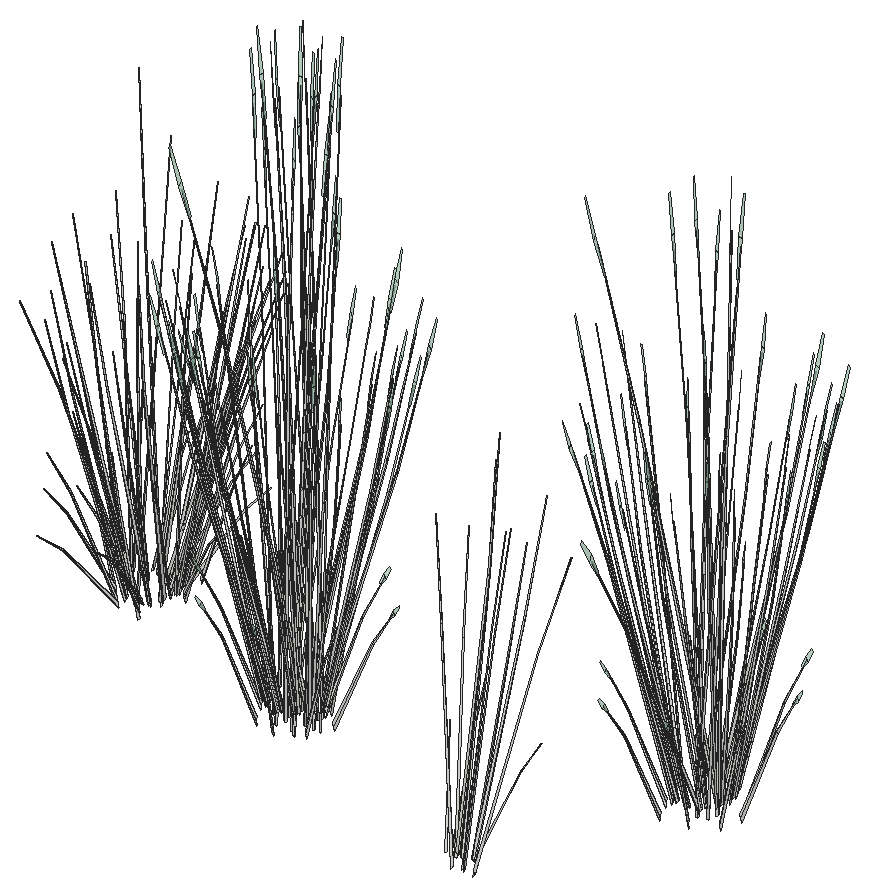
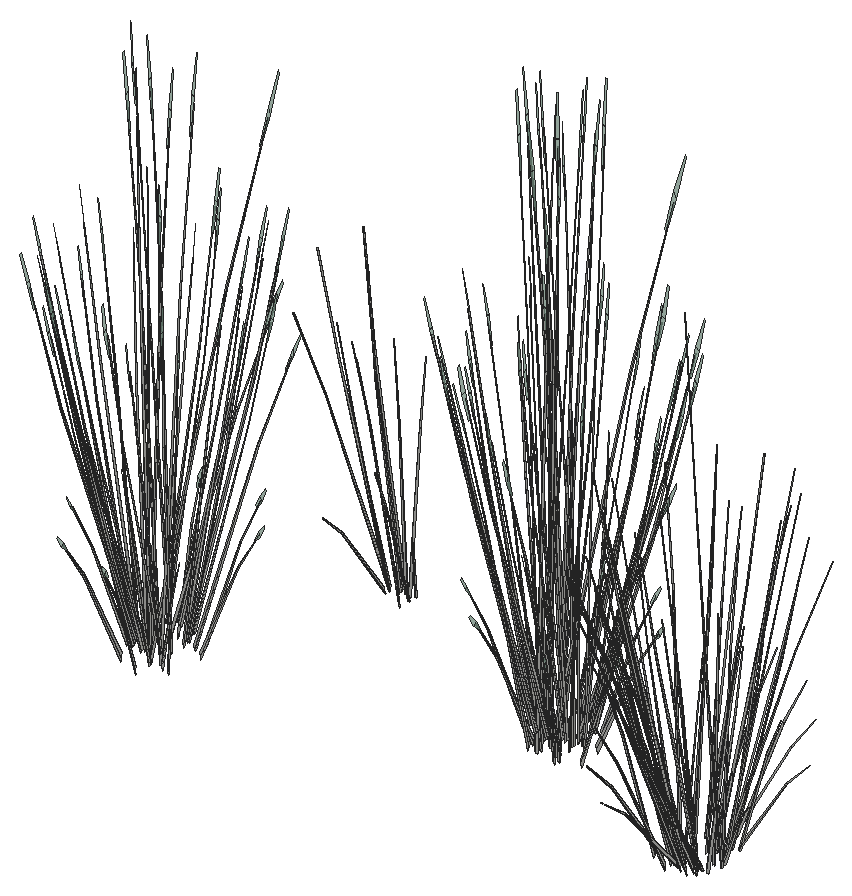
# SketchUp Ruby script. Lengths in inches.
U = 1.inch
M = Sketchup.active_model
def pt(a) = Geom::Point3d.new(a.map { |v| v * U })
def face(e, loops, mat)
  f = e.add_face(loops[0].map { |a| pt(a) })
  loops[1..].each { |l| e.add_face(l.map { |a| pt(a) }).erase! }
  f.material = f.back_material = mat if mat
  f
end
# faces: each face lists its corners as indices into pts; further lists are holes
def faces(e, pts, list, mat = nil) = list.each { |f| face(e, (f[0].is_a?(Array) ? f : [f]).map { |l| l.map { |i| pts[i] } }, mat) }
# xy, xz, yz: faces in a plane at the given z, y or x. An outline is a flat list of corners, or four numbers for a rectangle; further outlines are holes
def ring(l) = l.size == 4 ? [[l[0], l[1]], [l[2], l[1]], [l[2], l[3]], [l[0], l[3]]] : l.each_slice(2).to_a
def flat(e, list, mat, &to3) = list.each { |f| face(e, (f[0].is_a?(Array) ? f : [f]).map { |l| ring(l).map { |u, v| to3.(u, v) } }, mat) }
def xy(e, z, list, mat = nil) = flat(e, list, mat) { |x, y| [x, y, z] }
def xz(e, y, list, mat = nil) = flat(e, list, mat) { |x, z| [x, y, z] }
def yz(e, x, list, mat = nil) = flat(e, list, mat) { |y, z| [x, y, z] }
def lines(e, pts, list) = list.each { |a, b| e.add_line(pt(pts[a]), pt(pts[b])) }
# prism: a flat outline (further loops are holes) pulled along v
def prism(e, loops, v, mat = nil)
  f = face(e, loops, mat); d = Geom::Vector3d.new(v.map { |x| x * U })
  f.pushpull(f.normal.samedirection?(d) ? d.length : -d.length)
end
def box(e, o, s, mat = nil) = prism(e, [[o, [o[0] + s[0], o[1], o[2]], [o[0] + s[0], o[1] + s[1], o[2]], [o[0], o[1] + s[1], o[2]]]], [0, 0, s[2]], mat)
def at(x, y, z, deg = 0) = Geom::Transformation.translation(pt([x, y, z])) * Geom::Transformation.rotation(ORIGIN, Z_AXIS, deg.degrees)
def axes(o, x, y, z) = Geom::Transformation.new([*x, 0, *y, 0, *z, 0, *pt(o).to_a, 1])
def part(name) = M.definitions.add(name)
# library, detail: a bought-in or finely detailed component or shape, given as its bounding box
def library(name, o, s) = part(name).tap { |d| box(d.entities, o, s) }
def detail(e, o, s) = box(e.add_group.entities, o, s)
def put(e, d, t, mat = nil) = e.add_instance(d, t).tap { |i| i.material = mat if mat }
def group(e, t, mat = nil) = e.add_group.tap { |g| g.transformation = t; g.material = mat if mat }.entities
root = M.entities
M.materials.add("LightPink_Translucent").color = [175, 214, 192]
M.materials["LightPink_Translucent"].alpha = 0.75
c1 = part("blade")
p = [[2.15,0.21,22],[0,0.17,0],[0.09,0.45,0],[2.18,0.31,22],[2.29,0.31,22],[0.38,0.45,0],
  [2.48,0.24,33],[2.49,0.24,33],[2.48,0.22,33]]
faces(c1.entities,p,[[0,1,2,3],[4,5,2,3],[6,3,4,7],[8,0,3,6]])
c2 = part("blade with seeds\#1")
put(c2.entities,c1,at(0,0,0))
c3 = part("seeds")
p = [[0.3,-0.1,1.38],[-0.01,-0.03,1.59],[-0.01,-0.03,0.03],[0.14,-0.07,-0.07],[0.29,-0.03,3],[0.15,0.01,3.11]]
faces(c3.entities,p,[[0,1,2,3],[1,0,4,5]],"LightPink_Translucent")
c4 = part("blade with seeds")
put(c4.entities,c1,at(0,0,0))
put(c4.entities,c3,axes([2.4,0.25,30.99],[1.5799,-0.05474,1.17369],[-0.12525,1.92788,0.29478],[-0.07173,-0.02425,1.56792]))
put(root,c2,axes([484.5,550.33,139.9],[0.09256,-0.13097,1.40588],[0.38832,0.27104,0.11368],[-0.17518,0.16893,0.601]))
put(root,c2,axes([484.61,551.07,140.43],[-0.33637,0.20062,-0.29052],[-0.31842,-0.22908,0.37506],[-0.04845,0.11639,0.71765]))
put(root,c2,axes([483.45,551.01,140.59],[-0.01236,0.0754,1.43516],[0.35069,0.26232,-0.22697],[-0.09181,0.12405,0.1151]))
put(root,c2,axes([484.57,550.84,141.15],[0.54637,0.01888,-0.11073],[-0.01493,0.35746,-0.6146],[-0.03795,0.13767,0.93387]))
put(root,c2,axes([485.58,551.24,140.85],[0.48648,-0.17741,-0.09976],[0.23906,0.31487,-0.55369],[0.06419,0.13269,0.84132]))
put(root,c2,axes([484.94,550.98,140.82],[0.35588,0.25603,-0.4653],[-0.37594,0.22422,-0.36041],[-0.05415,0.13008,0.89031]))
put(root,c2,axes([486.28,550.55,139.9],[-0.11364,-0.12234,1.40588],[0.52511,-0.103,0.11368],[0.11868,0.19206,0.601]))
put(root,c2,axes([485.78,551.43,140.43],[-0.14987,0.29303,-0.29052],[-0.43725,-0.08547,0.37506],[0.04009,0.11798,0.71765]))
put(root,c2,axes([485.35,550.61,139.9],[-0.01217,-0.14625,1.40588],[0.52737,0.09702,0.11368],[-0.03262,0.20842,0.601]))
put(root,c2,axes([483.41,551.79,140.58],[0.0564,-0.02301,1.45516],[0.46615,0.15302,-0.1375],[-0.01095,0.12741,0.25751]))
put(root,c2,axes([485.47,551.95,140.59],[0.06302,0.06136,1.43516],[0.50855,0.02411,-0.22697],[0.05114,0.13532,0.1151]))
put(root,c2,axes([484.65,551.36,139.48],[0.01092,-0.19671,1.26617],[0.49126,0.1039,0.17497],[-0.04257,0.20964,0.59789]))
put(root,c4,axes([463.59,558.34,141.8],[-0.22811,-0.3621,-0.64651],[0.46957,-0.2018,0.07802],[-0.05334,-0.17496,0.91455]))
put(root,c4,axes([464.54,558.7,141.8],[0.01244,-0.41193,-0.64651],[0.52368,0.02767,0.07802],[0.05527,-0.17451,0.91455]))
put(root,c4,axes([463.63,558.04,141.38],[0.14409,-0.34247,-0.32227],[0.42037,0.09989,0.41605],[-0.03855,-0.13788,0.79608]))
put(root,c4,axes([463.42,558.27,141.52],[-0.46982,-0.11164,-0.465],[0.16104,-0.38276,-0.36018],[-0.04308,-0.1541,0.88973]))
put(root,c4,axes([463.71,557.3125,139.78],[0.06131,0.25968,1.04523],[-0.34012,-0.14383,0.76796],[0.0366,-0.13297,0.23022]))
put(root,c4,axes([464.43,558.56,141.52],[-0.34214,-0.29922,-0.465],[0.36143,-0.26205,-0.36018],[0.05206,-0.15203,0.88973]))
put(root,c4,axes([464.76,558.45,141.38],[0.32338,-0.23447,-0.32227],[0.30612,0.26773,0.41605],[0.04658,-0.13603,0.79608]))
put(root,c4,axes([461.96,557.625,139.78],[0.24931,0.155,1.04523],[-0.36309,0.09317,0.76796],[-0.07769,-0.11912,0.23022]))
put(root,c4,axes([462.5625,558.45,141.8],[-0.40754,-0.21525,-0.64651],[0.28963,-0.37719,0.07802],[-0.14765,-0.12852,0.91455]))
put(root,c4,axes([462.42,558.16,141.38],[-0.07382,-0.3587,-0.32227],[0.42197,-0.09472,0.41605],[-0.11334,-0.10279,0.79608]))
put(root,c4,axes([462.37,558.46,141.52],[-0.47162,0.10586,-0.465],[-0.0825,-0.4009,-0.36018],[-0.12667,-0.11489,0.88973]))
put(root,c4,axes([465.16,559.41,141.8],[0.24965,-0.35138,-0.64651],[0.43748,0.24972,0.07802],[0.14906,-0.12731,0.91455]))
put(root,c4,axes([465.14,559.25,141.52],[-0.12278,-0.40663,-0.465],[0.46497,-0.07113,-0.36018],[0.13325,-0.10922,0.88973]))
put(root,c4,axes([463.54,560.88,140.29],[0.41302,0.17958,1.37647],[-0.40462,0.38687,0.54432],[-0.18124,-0.22929,1.15394]))
put(root,c4,axes([465.71,558.44,139.78],[-0.15919,0.2267,1.04523],[-0.13683,-0.30457,0.76796],[0.13148,-0.07632,0.23022]))
put(root,c4,axes([465.49,559.29,141.38],[0.41603,-0.06364,-0.32227],[0.10985,0.36383,0.41605],[0.11922,-0.09772,0.79608]))
put(root,c4,axes([461.44,558.79,141.38],[-0.27194,-0.27882,-0.32227],[0.31051,-0.26394,0.41605],[-0.15777,-0.04016,0.79608]))
put(root,c4,axes([461.73,558.98,141.8],[-0.47777,-0.01072,-0.64651],[0.03209,-0.45152,0.07802],[-0.2024,-0.04765,0.91455]))
put(root,c4,axes([461.57,559.07,141.52],[-0.34704,0.29499,-0.465],[-0.30393,-0.31162,-0.36018],[-0.17633,-0.04488,0.88973]))
put(root,c4,axes([460.79,559.46,139.78],[0.30513,-0.03187,1.04523],[-0.19355,0.28077,0.76796],[-0.15079,-0.04212,0.23022]))
put(root,c4,axes([462.95,559.72,139.74],[-0.519,0.02749,0.40713],[-0.04694,-0.45634,-0.19594],[0.09291,-0.04625,1.30716]))
put(root,c4,axes([461.61,560.05,139.52],[0,0.44533,0.45182],[-0.53472,0,0],[0,-0.10143,1.43328]))
put(root,c4,axes([465.36,560.15,141.52],[0.12948,-0.40508,-0.465],[0.44393,0.13885,-0.36018],[0.17873,-0.03714,0.88973]))
put(root,c4,axes([462.82,560.28,139.74],[-0.23189,0.40128,0.40713],[-0.48183,-0.19312,-0.19594],[0,-0.0925,1.30716]))
put(root,c4,axes([464.4,558.74,139.52],[-0.44731,-0.22267,0.45182],[0.26736,-0.39927,0],[0.10188,0.05071,1.43328]))
put(root,c4,axes([465.28,560.3,141.8],[0.41997,-0.19668,-0.64651],[0.23405,0.40486,0.07802],[0.20292,-0.04599,0.91455]))
put(root,c4,axes([462.7,558.9375,139.52],[-0.13807,0.44258,0.16054],[-0.50524,-0.12525,0.31929],[0.08728,-0.00216,1.4597]))
put(root,c4,axes([463.57,559.53,139.74],[-0.28711,-0.37379,0.40713],[0.43489,-0.26322,-0.19594],[0.09291,0.04625,1.30716]))
put(root,c4,axes([462.66,561.22,139.52],[0.51358,-0.1182,0.16054],[0.12682,0.43988,0.31929],[-0.0458,-0.06409,1.4597]))
put(root,c4,axes([465.63,560.34,141.38],[0.3972,0.12423,-0.32227],[-0.11585,0.36244,0.41605],[0.15992,-0.03323,0.79608]))
put(root,c4,axes([460.96,559.76,141.38],[-0.3972,-0.12423,-0.32227],[0.11585,-0.36244,0.41605],[-0.15992,0.03323,0.79608]))
put(root,c4,axes([464.23,558.96,139.52],[-0.51358,0.1182,0.16054],[-0.12682,-0.43988,0.31929],[0.0458,0.06409,1.4597]))
put(root,c2,axes([445.41,563.42,140.68],[-0.05804,-0.06898,1.43516],[-0.35603,0.0883,-0.22697],[-0.0675,-0.17309,0.1151]))
put(root,c4,axes([464.18,561.24,139.52],[0.13807,-0.44258,0.16054],[0.50524,0.12525,0.31929],[-0.08728,0.00216,1.4597]))
put(root,c4,axes([462.17,559.7,140.31],[0.13585,-0.06442,1.61128],[0.04685,0.4498,0.1261],[-0.29426,0.05969,0.57588]))
put(root,c4,axes([464.97,560.11,139.52],[-0.37551,-0.32439,0.16054],[0.37842,-0.31463,0.31929],[-0.04147,0.06625,1.4597]))
put(root,c4,axes([466.47,560.41,139.78],[-0.2953,0.07352,1.04523],[0.139,-0.30384,0.76796],[0.15666,0.02079,0.23022]))
put(root,c2,axes([446.97,563.78,140.68],[-0.03336,0.04495,1.45516],[-0.35758,-0.09833,-0.1375],[-0.02285,-0.17707,0.25751]))
put(root,c4,axes([462.49,561.44,139.52],[0.44731,0.22267,0.45182],[-0.26736,0.39927,0],[-0.10188,-0.05071,1.43328]))
put(root,c2,axes([445.43,565.64,139.99],[0.00863,0.2062,1.40588],[-0.37404,-0.13679,0.11368],[0.02314,-0.29386,0.601]))
put(root,c4,axes([464.07,559.9,139.74],[0.23189,-0.40128,0.40713],[0.48183,0.19312,-0.19594],[0,0.0925,1.30716]))
put(root,c4,axes([461.24,559.94,141.52],[-0.12948,0.40508,-0.465],[-0.44393,-0.13885,-0.36018],[-0.17873,0.03714,0.88973]))
put(root,c4,axes([493.37,566.32,140.21],[0.06442,0.13585,1.61128],[-0.4498,0.04685,0.1261],[-0.05969,-0.29426,0.57588]))
put(root,c2,axes([445.81,564.52,140.53],[0.1063,-0.41315,-0.29052],[0.31012,0.1205,0.37506],[-0.02844,-0.16634,0.71765]))
put(root,c4,axes([465.28,560.125,139.52],[0,-0.44533,0.45182],[0.53472,0,0],[0,0.10143,1.43328]))
put(root,c4,axes([463.94,560.46,139.74],[0.519,-0.02749,0.40713],[0.04694,0.45634,-0.19594],[-0.09291,0.04625,1.30716]))
put(root,c4,axes([494.09,565.875,141.7],[0.01072,-0.47777,-0.64651],[0.45152,0.03209,0.07802],[0.04765,-0.2024,0.91455]))
put(root,c2,axes([446.43,564.9,140.68],[-0.00644,-0.10664,1.43516],[-0.29603,-0.29251,-0.22697],[0.03908,-0.18969,0.1151]))
put(root,c4,axes([493.3125,565.11,141.29],[0.12423,-0.3972,-0.32227],[0.36244,0.11585,0.41605],[-0.03323,-0.15992,0.79608]))
put(root,c4,axes([493.125,565.38,141.43],[-0.40508,-0.12948,-0.465],[0.13885,-0.44393,-0.36018],[-0.03714,-0.17873,0.88973]))
put(root,c2,axes([445.95,564.78,140.94],[-0.34504,0.25013,-0.09976],[-0.16956,-0.44394,-0.55369],[-0.04552,-0.18708,0.84132]))
put(root,c2,axes([446.66,565.34,140.94],[-0.38751,-0.02662,-0.09976],[0.01059,-0.50399,-0.55369],[0.02692,-0.19411,0.84132]))
put(root,c4,axes([494,565.71,141.43],[-0.29499,-0.34704,-0.465],[0.31162,-0.30393,-0.36018],[0.04488,-0.17633,0.88973]))
put(root,c2,axes([445.04,563.67,140.68],[-0.00289,0.06493,1.45516],[-0.31009,0.26964,-0.1375],[-0.10196,-0.10828,0.25751]))
put(root,c2,axes([444.92,564.67,140.53],[-0.05446,-0.43273,-0.29052],[0.31131,-0.11427,0.37506],[-0.08362,-0.12401,0.71765]))
put(root,c2,axes([446.64,565.02,140.53],[0.23857,-0.28286,-0.29052],[0.22584,0.32298,0.37506],[0.03436,-0.1641,0.71765]))
put(root,c4,axes([464.86,561.12,141.8],[0.47777,0.01072,-0.64651],[-0.03209,0.45152,0.07802],[0.2024,0.04765,0.91455]))
put(root,c4,axes([464.33,561.48,139.52],[0.44731,-0.22267,0.45182],[0.26736,0.39927,0],[-0.10188,0.05071,1.43328]))
put(root,c4,axes([491.39,564.5,139.6875],[0.20183,0.19918,1.04523],[-0.31952,0.0786,0.76796],[-0.05721,-0.14394,0.23022]))
put(root,c2,axes([446.03,566.03,139.99],[-0.06565,0.18466,1.40588],[-0.27542,-0.38215,0.11368],[0.12424,-0.23818,0.601]))
put(root,c4,axes([494.28,565.59,141.29],[0.27882,-0.27194,-0.32227],[0.26394,0.31051,0.41605],[0.04016,-0.15777,0.79608]))
put(root,c4,axes([492.27,565.25,141.29],[-0.06364,-0.41603,-0.32227],[0.36383,-0.10985,0.41605],[-0.09772,-0.11922,0.79608]))
put(root,c4,axes([460.36,561.68,139.78],[0.19918,-0.20183,1.04523],[0.0786,0.31952,0.76796],[-0.14394,0.05721,0.23022]))
put(root,c4,axes([465.15,561.3,141.38],[0.27194,0.27882,-0.32227],[-0.31051,0.26394,0.41605],[0.15777,0.04016,0.79608]))
put(root,c4,axes([461.11,560.8,141.38],[-0.41603,0.06364,-0.32227],[-0.10985,-0.36383,0.41605],[-0.11922,0.09772,0.79608]))
put(root,c4,axes([493.61,564.93,139.6875],[0.03187,0.30513,1.04523],[-0.28077,-0.19355,0.76796],[0.04212,-0.15079,0.23022]))
put(root,c2,axes([446.67,564.17,140.04],[-0.32031,0.09515,-0.02864],[-0.07364,-0.44972,-0.12987],[0.02031,-0.09391,0.42837]))
put(root,c2,axes([445.13,564.8,140.94],[-0.21011,0.45986,-0.09976],[-0.30427,-0.26493,-0.55369],[-0.10577,-0.12992,0.84132]))
put(root,c4,axes([464.83,561.46,139.78],[-0.2691,-0.12805,1.04523],[0.34747,-0.13011,0.76796],[0.09372,0.11021,0.23022]))
put(root,c4,axes([492.22,565.59,141.43],[-0.40663,0.12278,-0.465],[-0.07113,-0.46497,-0.36018],[-0.10922,-0.13325,0.88973]))
put(root,c2,axes([447.09,566.33,140.94],[-0.32616,-0.29624,-0.09976],[0.1879,-0.42901,-0.55369],[0.09215,-0.14913,0.84132]))
put(root,c4,axes([461.45,560.85,141.52],[0.12278,0.40663,-0.465],[-0.46497,0.07113,-0.36018],[-0.13325,0.10922,0.88973]))
put(root,c4,axes([494.625,566.7,141.7],[0.21525,-0.40754,-0.64651],[0.37719,0.28963,0.07802],[0.12852,-0.14765,0.91455]))
put(root,c4,axes([494.61,566.51,141.43],[-0.10586,-0.47162,-0.465],[0.4009,-0.0825,-0.36018],[0.11489,-0.12667,0.88973]))
put(root,c4,axes([464.18,560.02,139.85],[-0.01306,-0.4193,1.28558],[0.59089,0.10869,0.54432],[-0.13975,0.22943,1.21348]))
put(root,c2,axes([444.23,566.27,139.99],[0.13097,0.09256,1.40588],[-0.27104,0.38832,0.11368],[-0.16893,-0.17518,0.601]))
put(root,c4,axes([464.22,561.64,141.52],[0.47162,-0.10586,-0.465],[0.0825,0.4009,-0.36018],[0.12667,0.11489,0.88973]))
put(root,c4,axes([464.875,562.05,139.69],[-0.30649,-0.01397,0.95605],[0.2024,-0.29664,0.52785],[0.12108,0.10539,0.74993]))
put(root,c2,axes([443.86,564.9,140.68],[-0.07584,0.0048,1.43516],[-0.21918,0.40531,-0.22697],[-0.13286,-0.06266,0.1151]))
put(root,c2,axes([445.16,566,140.48],[-0.19798,0.42958,1.1344],[-0.30825,-0.45359,0.48946],[0.18577,-0.1386,1.09651]))
put(root,c2,axes([444.19,565.43,140.53],[-0.20062,-0.33637,-0.29052],[0.22908,-0.31842,0.37506],[-0.11639,-0.04845,0.71765]))
put(root,c2,axes([447.36,566.72,140.68],[-0.04613,-0.00147,1.45516],[-0.20353,-0.42603,-0.1375],[0.07265,-0.14798,0.25751]))
put(root,c4,axes([461.84,561.65,141.38],[-0.32338,0.23447,-0.32227],[-0.30612,-0.26773,0.41605],[-0.04658,0.13603,0.79608]))
put(root,c4,axes([494.91,566.5625,141.29],[0.3587,-0.07382,-0.32227],[0.09472,0.42197,0.41605],[0.10279,-0.11334,0.79608]))
put(root,c4,axes([462.05,562.56,139.78],[-0.01237,-0.2648,1.04523],[0.30908,0.18886,0.76796],[-0.06079,0.12621,0.23022]))
put(root,c4,axes([491.42,565.98,141.29],[-0.23447,-0.32338,-0.32227],[0.26773,-0.30612,0.41605],[-0.13603,-0.04658,0.79608]))
put(root,c4,axes([462.16,561.54,141.82],[0.34214,0.29922,-0.51615],[-0.36143,0.26205,-0.3998],[-0.05206,0.15203,0.9876]))
put(root,c2,axes([446.41,566.79,139.99],[-0.12234,0.11364,1.40588],[-0.103,-0.52511,0.11368],[0.19206,-0.11868,0.601]))
put(root,c4,axes([463.18,561.83,141.52],[0.46982,0.11164,-0.465],[-0.16104,0.38276,-0.36018],[0.04308,0.1541,0.88973]))
put(root,c4,axes([492.19,567.68,140.2],[-0.17958,0.41302,1.37647],[-0.38687,-0.40462,0.54432],[0.22929,-0.18124,1.15394]))
put(root,c4,axes([495.45,566.1,139.6875],[-0.155,0.24931,1.04523],[-0.09317,-0.36309,0.76796],[0.11912,-0.07769,0.23022]))
put(root,c4,axes([462.96,562.0625,141.38],[-0.14409,0.34247,-0.32227],[-0.42037,-0.09989,0.41605],[0.03855,0.13788,0.79608]))
put(root,c4,axes([491.67,566.2,142.03],[-0.41193,-0.01244,-0.71763],[0.02767,-0.52368,0.0866],[-0.17451,-0.05527,1.01516]))
put(root,c4,axes([490.51,566.1875,139.6875],[0.2648,-0.01237,1.04523],[-0.18886,0.30908,0.76796],[-0.12621,-0.06079,0.23022]))
put(root,c4,axes([462.06,561.4,142.125],[-0.01244,0.41193,-0.71763],[-0.52368,-0.02767,0.0866],[-0.05527,0.17451,1.01516]))
put(root,c4,axes([491.09,566.02,140.23],[0.22989,0.0105,1.40454],[-0.12143,0.4723,0.19409],[-0.24501,-0.04092,0.66323]))
put(root,c2,axes([444.42,565.39,140.94],[-0.01888,0.54637,-0.09976],[-0.35746,-0.01493,-0.55369],[-0.13767,-0.03795,0.84132]))
put(root,c4,axes([463.01,561.75,141.8],[0.22811,0.3621,-0.64651],[-0.46957,0.2018,0.07802],[0.05334,0.17496,0.91455]))
put(root,c2,axes([443.58,565,140.68],[0.0291,0.05049,1.45516],[-0.09819,0.49465,-0.1375],[-0.12701,0.01791,0.25751]))
put(root,c2,axes([447.1,567.49,140.94],[-0.17741,-0.48648,-0.09976],[0.31487,-0.23906,-0.55369],[0.13269,-0.06419,0.84132]))
put(root,c4,axes([491.54,566.3,141.72],[-0.29922,0.34214,-0.51615],[-0.26205,-0.36143,-0.3998],[-0.15203,-0.05206,0.9876]))
put(root,c4,axes([493.05,568.32,139.76],[0.4193,-0.01306,1.28558],[-0.10869,0.59089,0.54432],[-0.22943,-0.13975,1.21348]))
put(root,c4,axes([461.88,561.98,140.33],[0.0105,-0.22989,1.40454],[0.4723,0.12143,0.19409],[-0.04092,0.24501,0.66323]))
put(root,c4,axes([494.8,567.56,141.43],[0.11164,-0.46982,-0.465],[0.38276,0.16104,-0.36018],[0.1541,-0.04308,0.88973]))
put(root,c2,axes([447.8,567.6,140.68],[0.06136,-0.06302,1.43516],[0.02411,-0.50855,-0.22697],[0.13532,-0.05114,0.1151]))
put(root,c4,axes([492.79,566.97,139.64],[-0.40128,-0.23189,0.40713],[0.19312,-0.48183,-0.19594],[0.0925,0,1.30716]))
put(root,c4,axes([494.73,567.73,141.7],[0.3621,-0.22811,-0.64651],[0.2018,0.46957,0.07802],[0.17496,-0.05334,0.91455]))
put(root,c2,axes([443.84,566.6,140.53],[-0.29303,-0.14987,-0.29052],[0.08547,-0.43725,0.37506],[-0.11798,0.04009,0.71765]))
put(root,c2,axes([447.28,567.29,140.53],[0.29303,0.14987,-0.29052],[-0.08547,0.43725,0.37506],[0.11798,-0.04009,0.71765]))
put(root,c4,axes([492.61,568.08,139.64],[0.02749,0.519,0.40713],[-0.45634,0.04694,-0.19594],[-0.04625,-0.09291,1.30716]))
put(root,c4,axes([495.04,567.77,141.29],[0.34247,0.14409,-0.32227],[-0.09989,0.42037,0.41605],[0.13788,-0.03855,0.79608]))
put(root,c4,axes([491.01,567.11,141.29],[-0.34247,-0.14409,-0.32227],[0.09989,-0.42037,0.41605],[-0.13788,0.03855,0.79608]))
put(root,c4,axes([493.35,567.09,139.64],[-0.02749,-0.519,0.40713],[0.45634,-0.04694,-0.19594],[0.04625,0.09291,1.30716]))
put(root,c2,axes([446.47,567.72,139.99],[-0.14625,0.01217,1.40588],[0.09702,-0.52737,0.11368],[0.20842,0.03262,0.601]))
put(root,c2,axes([444.03,566.4,140.94],[0.17741,0.48648,-0.09976],[-0.31487,0.23906,-0.55369],[-0.13269,0.06419,0.84132]))
put(root,c4,axes([491.32,567.15,141.7],[-0.3621,0.22811,-0.64651],[-0.2018,-0.46957,0.07802],[-0.17496,0.05334,0.91455]))
put(root,c4,axes([495.76,567.85,139.6875],[-0.25968,0.06131,1.04523],[0.14383,-0.34012,0.76796],[0.13297,0.0366,0.23022]))
put(root,c4,axes([493.17,568.21,139.64],[0.40128,0.23189,0.40713],[-0.19312,0.48183,-0.19594],[-0.0925,0,1.30716]))
put(root,c2,axes([446.84,568.125,140.92],[0.25603,-0.35588,-0.4653],[0.22422,0.37594,-0.36041],[0.13008,0.05415,0.89031]))
put(root,c4,axes([491.25,567.32,141.43],[-0.11164,0.46982,-0.465],[-0.38276,-0.16104,-0.36018],[-0.1541,0.04308,0.88973]))
put(root,c2,axes([443.2,567.17,140.68],[-0.05342,0.07604,1.43516],[0.03387,0.50744,-0.22697],[-0.12778,0.08099,0.1151]))
put(root,c2,axes([447.21,568.42,139.57],[-0.19671,-0.01092,1.26617],[0.1039,-0.49126,0.17497],[0.20964,0.04257,0.59789]))
put(root,c4,axes([493.54,567.71,139.64],[0.37379,-0.28711,0.40713],[0.26322,0.43489,-0.19594],[-0.04625,0.09291,1.30716]))
put(root,c4,axes([494.51,568.58,141.43],[0.29922,-0.34214,-0.465],[0.26205,0.36143,-0.36018],[0.15203,0.05206,0.88973]))
put(root,c2,axes([446.72,568.24,141.19],[0.35246,0.01294,-0.64693],[-0.02367,0.54471,0.07807],[0.14932,0.05748,0.91515]))
put(root,c2,axes([446.27,566.7,139.54],[0.15365,-0.4296,1.24087],[0.33102,0.42086,0.4907],[-0.19619,0.18851,1.04025]))
put(root,c2,axes([447.64,569.66,140.68],[-0.02301,-0.0564,1.45516],[0.15302,-0.46615,-0.1375],[0.12741,0.01095,0.25751]))
put(root,c2,axes([443.95,567.86,140.53],[-0.30692,0.07678,-0.29052],[-0.08104,-0.43892,0.37506],[-0.08795,0.11789,0.71765]))
put(root,c2,axes([446.93,568.46,140.53],[0.20062,0.33637,-0.29052],[-0.22908,0.31842,0.37506],[0.11639,0.04845,0.71765]))
put(root,c4,axes([494.375,568.68,141.7],[0.41193,0.01244,-0.64651],[-0.02767,0.52368,0.07802],[0.17451,0.05527,0.91455]))
put(root,c2,axes([444.01,568.04,139.99],[0.12234,-0.11364,1.40588],[0.103,0.52511,0.11368],[-0.19206,0.11868,0.601]))
put(root,c2,axes([443.03,567.7,140.68],[0.04567,0.00927,1.45516],[0.16576,0.45742,-0.1375],[-0.08473,0.1346,0.25751]))
put(root,c4,axes([494.62,568.9,141.29],[0.23447,0.32338,-0.32227],[-0.26773,0.30612,0.41605],[0.13603,0.04658,0.79608]))
put(root,c4,axes([491.61,568.97,139.6875],[0.12805,-0.2691,1.04523],[0.13011,0.34747,0.76796],[-0.11021,0.09372,0.23022]))
put(root,c2,axes([446,569.09,140.94],[0.21011,-0.45986,-0.09976],[0.30427,0.26493,-0.55369],[0.10577,0.12992,0.84132]))
put(root,c4,axes([491.02,569.02,139.6],[0.01397,-0.30649,0.95605],[0.29664,0.2024,0.52785],[-0.10539,0.12108,0.74993]))
put(root,c2,axes([446.87,569.62,140.68],[0.0754,0.01236,1.43516],[0.26232,-0.35069,-0.22697],[0.12405,0.09181,0.1151]))
put(root,c2,axes([446.19,568.57,139.99],[-0.13097,-0.09256,1.40588],[0.27104,-0.38832,0.11368],[0.16893,0.17518,0.601]))
put(root,c4,axes([491.43,568.37,141.43],[0.10586,0.47162,-0.465],[-0.4009,0.0825,-0.36018],[-0.11489,0.12667,0.88973]))
put(root,c4,axes([493.82,569.29,141.43],[0.40663,-0.12278,-0.465],[0.07113,0.46497,-0.36018],[0.10922,0.13325,0.88973]))
put(root,c4,axes([491.72,570.1,140.75],[0.37435,-0.09148,-0.03177],[0.08606,0.43236,-0.14407],[-0.02373,0.09029,0.47519]))
put(root,c2,axes([445.9,568.48,139.99],[-0.11708,-0.12417,1.40588],[0.31602,-0.31352,0.11368],[0.14392,0.21504,0.601]))
put(root,c2,axes([444.49,568.875,140.53],[-0.23857,0.28286,-0.29052],[-0.22584,-0.32298,0.37506],[-0.03436,0.1641,0.71765]))
put(root,c2,axes([446.21,569.22,140.53],[0.05446,0.43273,-0.29052],[-0.31131,0.11427,0.37506],[0.08362,0.12401,0.71765]))
put(root,c2,axes([444.46,568.55,140.94],[0.38751,0.02662,-0.09976],[-0.01059,0.50399,-0.55369],[-0.02692,0.19411,0.84132]))
put(root,c4,axes([494.63,569.86,139.6875],[-0.2267,-0.15919,1.04523],[0.30457,-0.13683,0.76796],[0.07632,0.13148,0.23022]))
put(root,c2,axes([445.18,569.11,140.94],[0.34504,-0.25013,-0.09976],[0.16956,0.44394,-0.55369],[0.04552,0.18708,0.84132]))
put(root,c2,axes([443.79,568.84,140.68],[-0.00269,0.10696,1.43516],[0.26896,0.34054,-0.22697],[-0.05496,0.1817,0.1151]))
put(root,c2,axes([444.02,569.25,140.68],[0.03803,-0.03685,1.45516],[0.34183,0.17767,-0.1375],[0.00247,0.17994,0.25751]))
put(root,c4,axes([493.78,569.63,141.29],[0.06364,0.41603,-0.32227],[-0.36383,0.10985,0.41605],[0.09772,0.11922,0.79608]))
put(root,c4,axes([493.66,569.3,141.7],[0.35138,0.24965,-0.64651],[-0.24972,0.43748,0.07802],[0.12731,0.14906,0.91455]))
put(root,c4,axes([491.77,569.29,141.29],[-0.27882,0.27194,-0.32227],[-0.26394,-0.31051,0.41605],[-0.04016,0.15777,0.79608]))
put(root,c2,axes([445.89,570.54,140.68],[0.01022,-0.06344,1.45516],[0.33667,-0.19627,-0.1375],[0.08837,0.12987,0.25751]))
put(root,c2,axes([445.32,569.375,140.53],[-0.1063,0.41315,-0.29052],[-0.31012,-0.1205,0.37506],[0.02844,0.16634,0.71765]))
put(root,c2,axes([444.39,568.8,139.99],[0.06565,-0.18466,1.40588],[0.27542,0.38215,0.11368],[-0.12424,0.23818,0.601]))
put(root,c2,axes([445.52,569.63,140.68],[0.04947,0.08118,1.43516],[0.36146,-0.00691,-0.22697],[0.04701,0.18608,0.1151]))
put(root,c2,axes([445.26,568.12,139.55],[-0.05512,-0.14131,1.45254],[0.38487,-0.04873,0.11368],[0.05107,0.30608,0.51915]))
put(root,c4,axes([492.92,569.5,141.43],[0.40508,0.12948,-0.465],[-0.13885,0.44393,-0.36018],[0.03714,0.17873,0.88973]))
put(root,c4,axes([492.66,570.62,139.6875],[-0.07352,-0.2953,1.04523],[0.30384,0.139,0.76796],[-0.02079,0.15666,0.23022]))
put(root,c4,axes([492.73,569.77,141.29],[-0.12423,0.3972,-0.32227],[-0.36244,-0.11585,0.41605],[0.03323,0.15992,0.79608]))
put(root,c2,axes([445.65,569.11,139.99],[-0.0806,-0.17249,1.40588],[0.37244,-0.14522,0.11368],[0.08417,0.2708,0.601]))
put(root,c4,axes([491.95,569.01,141.7],[-0.01072,0.47777,-0.64651],[-0.45152,-0.03209,0.07802],[-0.04765,0.2024,0.91455]))
put(root,c4,axes([492.77,569.42,141.7],[0.19668,0.41997,-0.64651],[-0.40486,0.23405,0.07802],[0.04599,0.20292,0.91455]))
put(root,c2,axes([444.99,569.19,139.99],[-0.00863,-0.2062,1.40588],[0.37404,0.13679,0.11368],[-0.02314,0.29386,0.601]))
